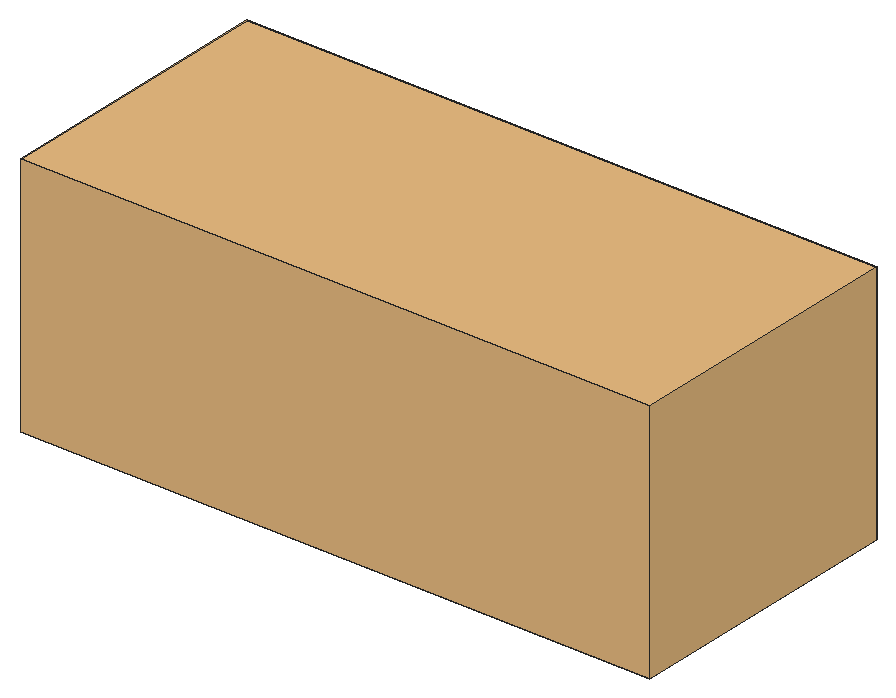
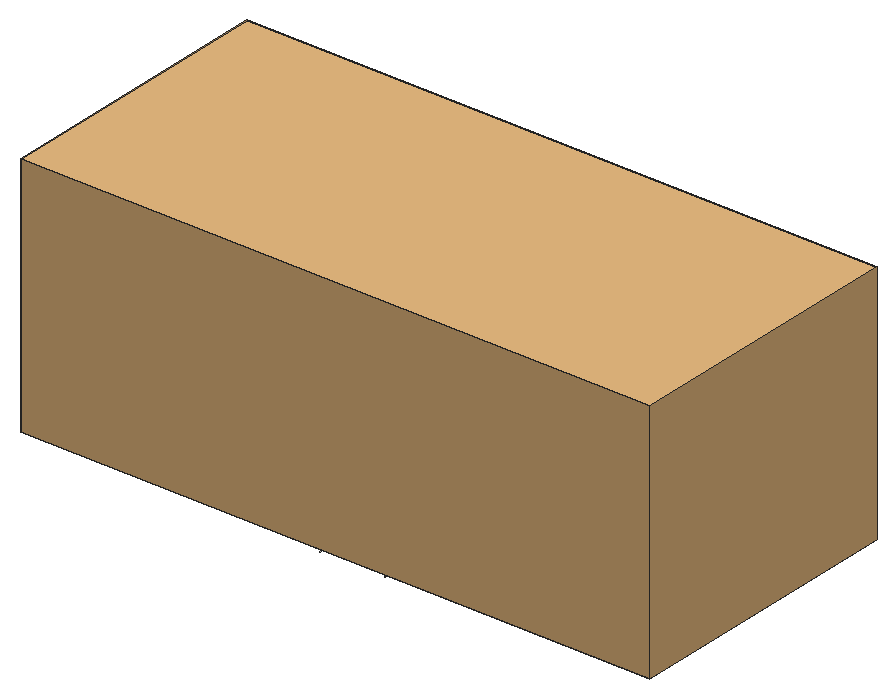
# SketchUp Ruby script. Lengths in inches.
U = 1.inch
M = Sketchup.active_model
def pt(a) = Geom::Point3d.new(a.map { |v| v * U })
def face(e, loops, mat)
  f = e.add_face(loops[0].map { |a| pt(a) })
  loops[1..].each { |l| e.add_face(l.map { |a| pt(a) }).erase! }
  f.material = f.back_material = mat if mat
  f
end
# faces: each face lists its corners as indices into pts; further lists are holes
def faces(e, pts, list, mat = nil) = list.each { |f| face(e, (f[0].is_a?(Array) ? f : [f]).map { |l| l.map { |i| pts[i] } }, mat) }
# xy, xz, yz: faces in a plane at the given z, y or x. An outline is a flat list of corners, or four numbers for a rectangle; further outlines are holes
def ring(l) = l.size == 4 ? [[l[0], l[1]], [l[2], l[1]], [l[2], l[3]], [l[0], l[3]]] : l.each_slice(2).to_a
def flat(e, list, mat, &to3) = list.each { |f| face(e, (f[0].is_a?(Array) ? f : [f]).map { |l| ring(l).map { |u, v| to3.(u, v) } }, mat) }
def xy(e, z, list, mat = nil) = flat(e, list, mat) { |x, y| [x, y, z] }
def xz(e, y, list, mat = nil) = flat(e, list, mat) { |x, z| [x, y, z] }
def yz(e, x, list, mat = nil) = flat(e, list, mat) { |y, z| [x, y, z] }
def lines(e, pts, list) = list.each { |a, b| e.add_line(pt(pts[a]), pt(pts[b])) }
# prism: a flat outline (further loops are holes) pulled along v
def prism(e, loops, v, mat = nil)
  f = face(e, loops, mat); d = Geom::Vector3d.new(v.map { |x| x * U })
  f.pushpull(f.normal.samedirection?(d) ? d.length : -d.length)
end
def box(e, o, s, mat = nil) = prism(e, [[o, [o[0] + s[0], o[1], o[2]], [o[0] + s[0], o[1] + s[1], o[2]], [o[0], o[1] + s[1], o[2]]]], [0, 0, s[2]], mat)
def at(x, y, z, deg = 0) = Geom::Transformation.translation(pt([x, y, z])) * Geom::Transformation.rotation(ORIGIN, Z_AXIS, deg.degrees)
def axes(o, x, y, z) = Geom::Transformation.new([*x, 0, *y, 0, *z, 0, *pt(o).to_a, 1])
def part(name) = M.definitions.add(name)
# library, detail: a bought-in or finely detailed component or shape, given as its bounding box
def library(name, o, s) = part(name).tap { |d| box(d.entities, o, s) }
def detail(e, o, s) = box(e.add_group.entities, o, s)
def put(e, d, t, mat = nil) = e.add_instance(d, t).tap { |i| i.material = mat if mat }
def group(e, t, mat = nil) = e.add_group.tap { |g| g.transformation = t; g.material = mat if mat }.entities
root = M.entities
M.materials.add("[Metal_Steel_Textured_White]").color = [191, 191, 191]
c1 = library("Land Rover Range Rover Sport",[-42.64,-96.16,0],[85.02,188.78,73.23])
xy(root,3.625,[[[147.359,164.396,134.847,169.578,143.617,178.348,148.799,165.836,148.641,165.764,148.487,165.682,148.339,165.59,148.198,165.489,148.063,165.378,147.936,165.259,147.817,165.132,147.706,164.998,147.605,164.856,147.513,164.708,147.431,164.555],[143.477,177.554,143.5,177.557,143.521,177.566,143.539,177.58,143.554,177.599,143.5625,177.62,143.566,177.643,143.5625,177.666,143.554,177.688,143.539,177.706,143.521,177.72,143.5,177.729,143.477,177.732,143.454,177.729,143.432,177.72,143.414,177.706,143.4,177.688,143.391,177.666,143.388,177.643,143.391,177.62,143.4,177.599,143.414,177.58,143.432,177.566,143.454,177.557],[139.514,173.592,139.537,173.595,139.559,173.604,139.577,173.618,139.591,173.637,139.6,173.658,139.603,173.681,139.6,173.704,139.591,173.725,139.577,173.744,139.559,173.758,139.537,173.767,139.514,173.77,139.491,173.767,139.47,173.758,139.451,173.744,139.4375,173.725,139.428,173.704,139.425,173.681,139.428,173.658,139.4375,173.637,139.451,173.618,139.47,173.604,139.491,173.595],[145.882,171.747,145.905,171.75,145.927,171.759,145.945,171.773,145.959,171.791,145.968,171.813,145.971,171.836,145.968,171.859,145.959,171.88,145.945,171.899,145.927,171.913,145.905,171.922,145.882,171.925,145.859,171.922,145.838,171.913,145.819,171.899,145.805,171.88,145.796,171.859,145.793,171.836,145.796,171.813,145.805,171.791,145.819,171.773,145.838,171.759,145.859,171.75],[141.495,175.573,141.518,175.576,141.54,175.585,141.558,175.599,141.572,175.618,141.581,175.639,141.584,175.662,141.581,175.685,141.572,175.707,141.558,175.725,141.54,175.739,141.518,175.748,141.495,175.751,141.472,175.748,141.451,175.739,141.433,175.725,141.418,175.707,141.41,175.685,141.407,175.662,141.41,175.639,141.418,175.618,141.433,175.599,141.451,175.585,141.472,175.576],[135.552,169.63,135.575,169.633,135.596,169.642,135.615,169.656,135.629,169.674,135.638,169.696,135.641,169.719,135.638,169.742,135.629,169.763,135.615,169.782,135.596,169.796,135.575,169.805,135.552,169.808,135.529,169.805,135.508,169.796,135.489,169.782,135.475,169.763,135.466,169.742,135.463,169.719,135.466,169.696,135.475,169.674,135.489,169.656,135.508,169.642,135.529,169.633],[148.288,165.939,148.311,165.942,148.332,165.951,148.351,165.965,148.365,165.984,148.374,166.005,148.377,166.028,148.374,166.051,148.365,166.073,148.351,166.091,148.332,166.105,148.311,166.114,148.288,166.117,148.265,166.114,148.243,166.105,148.225,166.091,148.211,166.073,148.202,166.051,148.199,166.028,148.202,166.005,148.211,165.984,148.225,165.965,148.243,165.951,148.265,165.942],[143.513,169.593,143.536,169.596,143.558,169.605,143.576,169.619,143.59,169.637,143.599,169.659,143.602,169.682,143.599,169.705,143.59,169.726,143.576,169.745,143.558,169.759,143.536,169.768,143.513,169.771,143.49,169.768,143.469,169.759,143.451,169.745,143.436,169.726,143.428,169.705,143.425,169.682,143.428,169.659,143.436,169.637,143.451,169.619,143.469,169.605,143.49,169.596],[137.533,171.611,137.556,171.614,137.578,171.623,137.596,171.637,137.61,171.655,137.619,171.677,137.622,171.7,137.619,171.723,137.61,171.744,137.596,171.763,137.578,171.777,137.556,171.786,137.533,171.789,137.51,171.786,137.489,171.777,137.47,171.763,137.456,171.744,137.447,171.723,137.444,171.7,137.447,171.677,137.456,171.655,137.47,171.637,137.489,171.623,137.51,171.614],[147.167,164.819,147.19,164.822,147.212,164.831,147.23,164.845,147.244,164.863,147.253,164.885,147.256,164.908,147.253,164.931,147.244,164.952,147.23,164.97,147.212,164.984,147.19,164.993,147.167,164.996,147.144,164.993,147.123,164.984,147.104,164.97,147.09,164.952,147.081,164.931,147.078,164.908,147.081,164.885,147.09,164.863,147.104,164.845,147.123,164.831,147.144,164.822],[144.679,174.651,144.702,174.654,144.724,174.663,144.742,174.677,144.756,174.695,144.765,174.717,144.768,174.74,144.765,174.763,144.756,174.784,144.742,174.802,144.724,174.817,144.702,174.825,144.679,174.828,144.656,174.825,144.635,174.817,144.617,174.802,144.602,174.784,144.594,174.763,144.591,174.74,144.594,174.717,144.602,174.695,144.617,174.677,144.635,174.663,144.656,174.654],[138.456,168.427,138.479,168.43,138.5,168.439,138.519,168.453,138.533,168.471,138.542,168.493,138.545,168.516,138.542,168.539,138.533,168.56,138.519,168.579,138.5,168.593,138.479,168.602,138.456,168.605,138.433,168.602,138.411,168.593,138.393,168.579,138.379,168.56,138.37,168.539,138.367,168.516,138.37,168.493,138.379,168.471,138.393,168.453,138.411,168.439,138.433,168.43],[141.36,167.224,141.383,167.227,141.404,167.236,141.422,167.25,141.437,167.269,141.445,167.29,141.448,167.313,141.445,167.336,141.437,167.358,141.422,167.376,141.404,167.39,141.383,167.399,141.36,167.402,141.337,167.399,141.315,167.39,141.297,167.376,141.283,167.358,141.274,167.336,141.271,167.313,141.274,167.29,141.283,167.269,141.297,167.25,141.315,167.236,141.337,167.227],[147.085,168.843,147.108,168.846,147.129,168.855,147.148,168.869,147.162,168.888,147.171,168.909,147.174,168.932,147.171,168.955,147.162,168.976,147.148,168.995,147.129,169.009,147.108,169.018,147.085,169.021,147.062,169.018,147.041,169.009,147.022,168.995,147.008,168.976,146.999,168.955,146.996,168.932,146.999,168.909,147.008,168.888,147.022,168.869,147.041,168.855,147.062,168.846],[144.263,166.021,144.286,166.024,144.308,166.033,144.326,166.047,144.34,166.066,144.349,166.087,144.352,166.11,144.349,166.133,144.34,166.155,144.326,166.173,144.308,166.187,144.286,166.196,144.263,166.199,144.24,166.196,144.219,166.187,144.2,166.173,144.186,166.155,144.177,166.133,144.174,166.11,144.177,166.087,144.186,166.066,144.2,166.047,144.219,166.033,144.24,166.024]],[[128.792,164.996,128.783,164.997,128.774,165.001,128.767,165.007,128.761,165.015,128.757,165.023,128.756,165.033,128.757,165.042,128.761,165.051,128.767,165.059,128.774,165.065,128.783,165.068,128.792,165.069,128.802,165.068,128.811,165.065,128.818,165.059,128.824,165.051,128.828,165.042,128.829,165.033,128.828,165.023,128.824,165.015,128.818,165.007,128.811,165.001,128.802,164.997],[128.792,165.013,128.798,165.014,128.802,165.016,128.807,165.019,128.81,165.023,128.812,165.028,128.8125,165.033,128.812,165.038,128.81,165.043,128.807,165.047,128.802,165.05,128.798,165.052,128.792,165.053,128.787,165.052,128.782,165.05,128.778,165.047,128.775,165.043,128.773,165.038,128.772,165.033,128.773,165.028,128.775,165.023,128.778,165.019,128.782,165.016,128.787,165.014]],[128.792,165.013,128.787,165.014,128.782,165.016,128.778,165.019,128.775,165.023,128.773,165.028,128.772,165.033,128.773,165.038,128.775,165.043,128.778,165.047,128.782,165.05,128.787,165.052,128.792,165.053,128.798,165.052,128.802,165.05,128.807,165.047,128.81,165.043,128.812,165.038,128.8125,165.033,128.812,165.028,128.81,165.023,128.807,165.019,128.802,165.016,128.798,165.014],[[148.799,165.836,143.617,178.348,156.019,178.348,150.836,165.836,150.673,165.898,150.507,165.948,150.337,165.988,150.165,166.016,149.992,166.033,149.818,166.039,149.644,166.033,149.471,166.016,149.299,165.988,149.129,165.948,148.962,165.898],[149.818,172.204,149.841,172.207,149.862,172.216,149.881,172.23,149.895,172.249,149.904,172.27,149.907,172.293,149.904,172.316,149.895,172.338,149.881,172.356,149.862,172.37,149.841,172.379,149.818,172.382,149.795,172.379,149.773,172.37,149.755,172.356,149.741,172.338,149.732,172.316,149.729,172.293,149.732,172.27,149.741,172.249,149.755,172.23,149.773,172.216,149.795,172.207],[154.219,174.956,154.242,174.959,154.263,174.968,154.282,174.982,154.296,175.001,154.305,175.022,154.308,175.045,154.305,175.068,154.296,175.09,154.282,175.108,154.263,175.122,154.242,175.131,154.219,175.134,154.196,175.131,154.174,175.122,154.156,175.108,154.142,175.09,154.133,175.068,154.13,175.045,154.133,175.022,154.142,175.001,154.156,174.982,154.174,174.968,154.196,174.959],[155.421,177.86,155.444,177.863,155.466,177.872,155.484,177.886,155.498,177.904,155.507,177.926,155.51,177.949,155.507,177.972,155.498,177.993,155.484,178.012,155.466,178.026,155.444,178.035,155.421,178.038,155.398,178.035,155.377,178.026,155.359,178.012,155.345,177.993,155.336,177.972,155.333,177.949,155.336,177.926,155.345,177.904,155.359,177.886,155.377,177.872,155.398,177.863],[144.214,177.86,144.237,177.863,144.259,177.872,144.277,177.886,144.291,177.904,144.3,177.926,144.303,177.949,144.3,177.972,144.291,177.993,144.277,178.012,144.259,178.026,144.237,178.035,144.214,178.038,144.191,178.035,144.17,178.026,144.151,178.012,144.137,177.993,144.128,177.972,144.125,177.949,144.128,177.926,144.137,177.904,144.151,177.886,144.17,177.872,144.191,177.863],[153.016,172.052,153.039,172.055,153.06,172.064,153.079,172.078,153.093,172.097,153.102,172.118,153.105,172.141,153.102,172.164,153.093,172.186,153.079,172.204,153.06,172.218,153.039,172.227,153.016,172.23,152.993,172.227,152.971,172.218,152.953,172.204,152.939,172.186,152.93,172.164,152.927,172.141,152.93,172.118,152.939,172.097,152.953,172.078,152.971,172.064,152.993,172.055],[147.016,177.86,147.039,177.863,147.061,177.872,147.079,177.886,147.093,177.904,147.102,177.926,147.105,177.949,147.102,177.972,147.093,177.993,147.079,178.012,147.061,178.026,147.039,178.035,147.016,178.038,146.993,178.035,146.972,178.026,146.953,178.012,146.939,177.993,146.93,177.972,146.927,177.949,146.93,177.926,146.939,177.904,146.953,177.886,146.972,177.872,146.993,177.863],[152.62,177.86,152.643,177.863,152.664,177.872,152.683,177.886,152.697,177.904,152.706,177.926,152.709,177.949,152.706,177.972,152.697,177.993,152.683,178.012,152.664,178.026,152.643,178.035,152.62,178.038,152.597,178.035,152.575,178.026,152.557,178.012,152.543,177.993,152.534,177.972,152.531,177.949,152.534,177.926,152.543,177.904,152.557,177.886,152.575,177.872,152.597,177.863],[145.417,174.956,145.44,174.959,145.462,174.968,145.48,174.982,145.494,175.001,145.503,175.022,145.506,175.045,145.503,175.068,145.494,175.09,145.48,175.108,145.462,175.122,145.44,175.131,145.417,175.134,145.394,175.131,145.373,175.122,145.354,175.108,145.34,175.09,145.331,175.068,145.328,175.045,145.331,175.022,145.34,175.001,145.354,174.982,145.373,174.968,145.394,174.959],[149.818,177.86,149.841,177.863,149.862,177.872,149.881,177.886,149.895,177.904,149.904,177.926,149.907,177.949,149.904,177.972,149.895,177.993,149.881,178.012,149.862,178.026,149.841,178.035,149.818,178.038,149.795,178.035,149.773,178.026,149.755,178.012,149.741,177.993,149.732,177.972,149.729,177.949,149.732,177.926,149.741,177.904,149.755,177.886,149.773,177.872,149.795,177.863],[147.823,169.149,147.846,169.152,147.867,169.161,147.886,169.175,147.9,169.193,147.909,169.215,147.912,169.238,147.909,169.261,147.9,169.282,147.886,169.3,147.867,169.315,147.846,169.323,147.823,169.326,147.8,169.323,147.778,169.315,147.76,169.3,147.746,169.282,147.737,169.261,147.734,169.238,147.737,169.215,147.746,169.193,147.76,169.175,147.778,169.161,147.8,169.152],[151.813,169.149,151.836,169.152,151.858,169.161,151.876,169.175,151.89,169.193,151.899,169.215,151.902,169.238,151.899,169.261,151.89,169.282,151.876,169.3,151.858,169.315,151.836,169.323,151.813,169.326,151.79,169.323,151.769,169.315,151.75,169.3,151.736,169.282,151.727,169.261,151.724,169.238,151.727,169.215,151.736,169.193,151.75,169.175,151.769,169.161,151.79,169.152],[146.62,172.052,146.643,172.055,146.664,172.064,146.683,172.078,146.697,172.097,146.706,172.118,146.709,172.141,146.706,172.164,146.697,172.186,146.683,172.204,146.664,172.218,146.643,172.227,146.62,172.23,146.597,172.227,146.575,172.218,146.557,172.204,146.543,172.186,146.534,172.164,146.531,172.141,146.534,172.118,146.543,172.097,146.557,172.078,146.575,172.064,146.597,172.055],[149.025,166.245,149.048,166.248,149.07,166.257,149.088,166.271,149.102,166.289,149.111,166.311,149.114,166.334,149.111,166.357,149.102,166.378,149.088,166.397,149.07,166.411,149.048,166.42,149.025,166.423,149.002,166.42,148.981,166.411,148.963,166.397,148.948,166.378,148.94,166.357,148.937,166.334,148.94,166.311,148.948,166.289,148.963,166.271,148.981,166.257,149.002,166.248],[150.61,166.245,150.633,166.248,150.655,166.257,150.673,166.271,150.6875,166.289,150.696,166.311,150.699,166.334,150.696,166.357,150.6875,166.378,150.673,166.397,150.655,166.411,150.633,166.42,150.61,166.423,150.587,166.42,150.566,166.411,150.547,166.397,150.533,166.378,150.524,166.357,150.521,166.334,150.524,166.311,150.533,166.289,150.547,166.271,150.566,166.257,150.587,166.248]],[[144.263,166.021,144.24,166.024,144.219,166.033,144.2,166.047,144.186,166.066,144.177,166.087,144.174,166.11,144.177,166.133,144.186,166.155,144.2,166.173,144.219,166.187,144.24,166.196,144.263,166.199,144.286,166.196,144.308,166.187,144.326,166.173,144.34,166.155,144.349,166.133,144.352,166.11,144.349,166.087,144.34,166.066,144.326,166.047,144.308,166.033,144.286,166.024],[144.263,166.022,144.286,166.025,144.307,166.034,144.326,166.048,144.339,166.066,144.348,166.088,144.351,166.11,144.348,166.133,144.339,166.154,144.326,166.172,144.307,166.186,144.286,166.195,144.263,166.198,144.241,166.195,144.219,166.186,144.201,166.172,144.187,166.154,144.178,166.133,144.175,166.11,144.178,166.088,144.187,166.066,144.201,166.048,144.219,166.034,144.241,166.025]],
  [[144.263,166.022,144.241,166.025,144.219,166.034,144.201,166.048,144.187,166.066,144.178,166.088,144.175,166.11,144.178,166.133,144.187,166.154,144.201,166.172,144.219,166.186,144.241,166.195,144.263,166.198,144.286,166.195,144.307,166.186,144.326,166.172,144.339,166.154,144.348,166.133,144.351,166.11,144.348,166.088,144.339,166.066,144.326,166.048,144.307,166.034,144.286,166.025],[144.263,166.074,144.273,166.075,144.282,166.079,144.289,166.084,144.295,166.092,144.299,166.101,144.3,166.11,144.299,166.12,144.295,166.129,144.289,166.136,144.282,166.142,144.273,166.146,144.263,166.147,144.254,166.146,144.245,166.142,144.237,166.136,144.232,166.129,144.228,166.12,144.227,166.11,144.228,166.101,144.232,166.092,144.237,166.084,144.245,166.079,144.254,166.075]],[[135.246,166.09,135.223,166.093,135.202,166.102,135.184,166.116,135.169,166.135,135.161,166.156,135.158,166.179,135.161,166.202,135.169,166.224,135.184,166.242,135.202,166.256,135.223,166.265,135.246,166.268,135.269,166.265,135.291,166.256,135.309,166.242,135.323,166.224,135.332,166.202,135.335,166.179,135.332,166.156,135.323,166.135,135.309,166.116,135.291,166.102,135.269,166.093],[135.246,166.091,135.269,166.094,135.29,166.103,135.309,166.117,135.323,166.135,135.331,166.156,135.334,166.179,135.331,166.202,135.323,166.223,135.309,166.241,135.29,166.255,135.269,166.264,135.246,166.267,135.224,166.264,135.202,166.255,135.184,166.241,135.17,166.223,135.161,166.202,135.159,166.179,135.161,166.156,135.17,166.135,135.184,166.117,135.202,166.103,135.224,166.094]],[[135.246,166.143,135.237,166.144,135.228,166.148,135.221,166.153,135.215,166.161,135.211,166.17,135.21,166.179,135.211,166.189,135.215,166.198,135.221,166.205,135.228,166.211,135.237,166.215,135.246,166.216,135.256,166.215,135.265,166.211,135.272,166.205,135.278,166.198,135.282,166.189,135.283,166.179,135.282,166.17,135.278,166.161,135.272,166.153,135.265,166.148,135.256,166.144],[135.246,166.159,135.252,166.16,135.256,166.162,135.261,166.165,135.264,166.169,135.266,166.174,135.266,166.184,135.264,166.189,135.261,166.193,135.256,166.197,135.252,166.198,135.246,166.199,135.236,166.197,135.232,166.193,135.229,166.189,135.227,166.184,135.226,166.179,135.227,166.174,135.229,166.169,135.232,166.165,135.236,166.162,135.241,166.16]],[135.246,166.159,135.241,166.16,135.236,166.162,135.232,166.165,135.229,166.169,135.227,166.174,135.226,166.179,135.227,166.184,135.229,166.189,135.232,166.193,135.236,166.197,135.246,166.199,135.252,166.198,135.256,166.197,135.261,166.193,135.264,166.189,135.266,166.184,135.266,166.174,135.264,166.169,135.261,166.165,135.256,166.162,135.252,166.16],[[134.448,166.256,134.425,166.259,134.404,166.268,134.385,166.282,134.371,166.3,134.362,166.322,134.359,166.345,134.362,166.368,134.371,166.389,134.385,166.407,134.404,166.422,134.425,166.43,134.448,166.433,134.471,166.43,134.492,166.422,134.511,166.407,134.525,166.389,134.534,166.368,134.537,166.345,134.534,166.322,134.525,166.3,134.511,166.282,134.492,166.268,134.471,166.259],[134.448,166.257,134.471,166.26,134.492,166.268,134.51,166.282,134.524,166.301,134.533,166.322,134.536,166.345,134.533,166.367,134.524,166.389,134.51,166.407,134.492,166.421,134.471,166.43,134.448,166.433,134.425,166.43,134.404,166.421,134.386,166.407,134.372,166.389,134.363,166.367,134.36,166.345,134.363,166.322,134.372,166.301,134.386,166.282,134.404,166.268,134.425,166.26]],
  [[134.448,166.308,134.439,166.309,134.43,166.313,134.422,166.319,134.416,166.326,134.413,166.335,134.411,166.345,134.413,166.354,134.416,166.363,134.422,166.37,134.43,166.376,134.439,166.38,134.448,166.381,134.457,166.38,134.466,166.376,134.474,166.37,134.48,166.363,134.483,166.354,134.485,166.345,134.483,166.335,134.48,166.326,134.474,166.319,134.466,166.313,134.457,166.309],[134.443,166.325,134.453,166.325,134.458,166.327,134.462,166.33,134.465,166.335,134.467,166.339,134.468,166.345,134.467,166.35,134.465,166.355,134.462,166.359,134.458,166.362,134.453,166.364,134.448,166.365,134.443,166.364,134.438,166.362,134.434,166.359,134.431,166.355,134.429,166.35,134.428,166.345,134.429,166.339,134.431,166.335,134.434,166.33,134.438,166.327]],[134.443,166.325,134.438,166.327,134.434,166.33,134.431,166.335,134.429,166.339,134.428,166.345,134.429,166.35,134.431,166.355,134.434,166.359,134.438,166.362,134.443,166.364,134.448,166.365,134.453,166.364,134.458,166.362,134.462,166.359,134.465,166.355,134.467,166.35,134.468,166.345,134.467,166.339,134.465,166.335,134.462,166.33,134.458,166.327,134.453,166.325],[[141.054,166.487,141.031,166.49,141.01,166.498,140.991,166.513,140.977,166.531,140.968,166.552,140.965,166.575,140.968,166.598,140.977,166.62,140.991,166.638,141.01,166.652,141.031,166.661,141.054,166.664,141.077,166.661,141.098,166.652,141.117,166.638,141.131,166.62,141.14,166.598,141.143,166.575,141.14,166.552,141.131,166.531,141.117,166.513,141.098,166.498,141.077,166.49],[141.054,166.488,141.077,166.491,141.098,166.499,141.116,166.513,141.13,166.531,141.139,166.553,141.142,166.575,141.139,166.598,141.13,166.619,141.116,166.638,141.098,166.652,141.077,166.66,141.054,166.663,141.031,166.66,141.01,166.652,140.992,166.638,140.978,166.619,140.969,166.598,140.966,166.575,140.969,166.553,140.978,166.531,140.992,166.513,141.01,166.499,141.031,166.491]],[[123.81,166.578,123.787,166.581,123.765,166.59,123.747,166.604,123.733,166.623,123.724,166.644,123.721,166.667,123.724,166.69,123.733,166.712,123.747,166.73,123.765,166.744,123.787,166.753,123.81,166.756,123.833,166.753,123.854,166.744,123.873,166.73,123.887,166.712,123.896,166.69,123.899,166.667,123.896,166.644,123.887,166.623,123.873,166.604,123.854,166.59,123.833,166.581],[123.81,166.579,123.833,166.582,123.854,166.591,123.872,166.605,123.886,166.623,123.895,166.644,123.898,166.667,123.895,166.69,123.886,166.711,123.872,166.729,123.854,166.743,123.833,166.752,123.81,166.755,123.787,166.752,123.766,166.743,123.748,166.729,123.734,166.711,123.725,166.69,123.722,166.667,123.725,166.644,123.734,166.623,123.748,166.605,123.766,166.591,123.787,166.582]],[[123.81,166.631,123.8,166.632,123.792,166.636,123.784,166.641,123.778,166.649,123.774,166.658,123.773,166.667,123.774,166.677,123.778,166.686,123.784,166.693,123.792,166.699,123.8,166.703,123.81,166.704,123.819,166.703,123.828,166.699,123.836,166.693,123.841,166.686,123.845,166.677,123.846,166.667,123.845,166.658,123.841,166.649,123.836,166.641,123.828,166.636,123.819,166.632],[123.81,166.647,123.815,166.648,123.82,166.65,123.824,166.653,123.827,166.657,123.829,166.662,123.83,166.667,123.829,166.672,123.827,166.677,123.824,166.681,123.82,166.685,123.815,166.687,123.805,166.687,123.8,166.685,123.796,166.681,123.793,166.677,123.791,166.672,123.79,166.667,123.791,166.662,123.793,166.657,123.796,166.653,123.8,166.65,123.805,166.648]],
  [123.81,166.647,123.805,166.648,123.8,166.65,123.796,166.653,123.793,166.657,123.791,166.662,123.79,166.667,123.791,166.672,123.793,166.677,123.796,166.681,123.8,166.685,123.805,166.687,123.815,166.687,123.82,166.685,123.824,166.681,123.827,166.677,123.829,166.672,123.83,166.667,123.829,166.662,123.827,166.657,123.824,166.653,123.82,166.65,123.815,166.648],[[141.36,167.224,141.337,167.227,141.315,167.236,141.297,167.25,141.283,167.269,141.274,167.29,141.271,167.313,141.274,167.336,141.283,167.358,141.297,167.376,141.315,167.39,141.337,167.399,141.36,167.402,141.383,167.399,141.404,167.39,141.422,167.376,141.437,167.358,141.445,167.336,141.448,167.313,141.445,167.29,141.437,167.269,141.422,167.25,141.404,167.236,141.383,167.227],[141.36,167.225,141.382,167.228,141.404,167.237,141.422,167.251,141.436,167.269,141.444,167.29,141.447,167.313,141.444,167.336,141.436,167.357,141.422,167.375,141.404,167.389,141.382,167.398,141.36,167.401,141.337,167.398,141.316,167.389,141.297,167.375,141.283,167.357,141.275,167.336,141.272,167.313,141.275,167.29,141.283,167.269,141.297,167.251,141.316,167.237,141.337,167.228]],[[141.36,167.276,141.35,167.278,141.341,167.281,141.334,167.287,141.328,167.295,141.324,167.304,141.323,167.313,141.324,167.323,141.328,167.331,141.334,167.339,141.341,167.345,141.35,167.348,141.36,167.35,141.369,167.348,141.378,167.345,141.385,167.339,141.391,167.331,141.395,167.323,141.396,167.313,141.395,167.304,141.391,167.295,141.385,167.287,141.378,167.281,141.369,167.278],[141.36,167.293,141.365,167.294,141.37,167.296,141.374,167.299,141.377,167.303,141.379,167.308,141.38,167.313,141.379,167.318,141.377,167.323,141.374,167.327,141.37,167.33,141.365,167.332,141.36,167.333,141.354,167.332,141.35,167.33,141.345,167.327,141.342,167.323,141.34,167.318,141.34,167.308,141.342,167.303,141.345,167.299,141.35,167.296,141.354,167.294]],[141.36,167.293,141.354,167.294,141.35,167.296,141.345,167.299,141.342,167.303,141.34,167.308,141.34,167.318,141.342,167.323,141.345,167.327,141.35,167.33,141.354,167.332,141.36,167.333,141.365,167.332,141.37,167.33,141.374,167.327,141.377,167.323,141.379,167.318,141.38,167.313,141.379,167.308,141.377,167.303,141.374,167.299,141.37,167.296,141.365,167.294],[[138.15,167.689,138.127,167.692,138.106,167.701,138.087,167.715,138.073,167.734,138.064,167.755,138.061,167.778,138.064,167.801,138.073,167.823,138.087,167.841,138.106,167.855,138.127,167.864,138.15,167.867,138.173,167.864,138.195,167.855,138.213,167.841,138.227,167.823,138.236,167.801,138.239,167.778,138.236,167.755,138.227,167.734,138.213,167.715,138.195,167.701,138.173,167.692],[138.15,167.69,138.173,167.693,138.194,167.702,138.212,167.716,138.226,167.734,138.235,167.755,138.238,167.778,138.235,167.801,138.226,167.822,138.212,167.84,138.194,167.854,138.173,167.863,138.15,167.866,138.127,167.863,138.106,167.854,138.088,167.84,138.074,167.822,138.065,167.801,138.062,167.778,138.065,167.755,138.074,167.734,138.088,167.716,138.106,167.702,138.127,167.693]],
  [[138.15,167.742,138.141,167.743,138.132,167.747,138.124,167.752,138.119,167.76,138.115,167.769,138.114,167.778,138.115,167.788,138.119,167.797,138.124,167.804,138.132,167.81,138.141,167.814,138.15,167.815,138.16,167.814,138.169,167.81,138.176,167.804,138.182,167.797,138.186,167.788,138.187,167.778,138.186,167.769,138.182,167.76,138.176,167.752,138.169,167.747,138.16,167.743],[138.15,167.758,138.155,167.759,138.16,167.761,138.164,167.764,138.168,167.768,138.17,167.778,138.168,167.788,138.16,167.796,138.155,167.798,138.145,167.798,138.14,167.796,138.136,167.792,138.133,167.788,138.131,167.783,138.13,167.778,138.131,167.773,138.133,167.768,138.136,167.764,138.14,167.761,138.145,167.759]],[138.15,167.758,138.145,167.759,138.14,167.761,138.136,167.764,138.133,167.768,138.131,167.773,138.13,167.778,138.131,167.783,138.133,167.788,138.136,167.792,138.14,167.796,138.145,167.798,138.155,167.798,138.16,167.796,138.168,167.788,138.17,167.778,138.168,167.768,138.164,167.764,138.16,167.761,138.155,167.759],[[128.792,168.255,128.769,168.258,128.748,168.267,128.73,168.281,128.715,168.299,128.707,168.321,128.704,168.344,128.707,168.367,128.715,168.388,128.73,168.406,128.748,168.421,128.769,168.429,128.792,168.432,128.815,168.429,128.837,168.421,128.855,168.406,128.869,168.388,128.878,168.367,128.881,168.344,128.878,168.321,128.869,168.299,128.855,168.281,128.837,168.267,128.815,168.258],[128.792,168.256,128.815,168.259,128.836,168.267,128.855,168.281,128.869,168.3,128.877,168.321,128.88,168.344,128.877,168.366,128.869,168.388,128.855,168.406,128.836,168.42,128.815,168.429,128.792,168.432,128.77,168.429,128.748,168.42,128.73,168.406,128.716,168.388,128.707,168.366,128.704,168.344,128.707,168.321,128.716,168.3,128.73,168.281,128.748,168.267,128.77,168.259]],[[128.792,168.307,128.783,168.308,128.774,168.312,128.767,168.318,128.761,168.325,128.757,168.334,128.756,168.344,128.757,168.353,128.761,168.362,128.767,168.369,128.774,168.375,128.783,168.379,128.792,168.38,128.802,168.379,128.811,168.375,128.818,168.369,128.824,168.362,128.828,168.353,128.829,168.344,128.828,168.334,128.824,168.325,128.818,168.318,128.811,168.312,128.802,168.308],[128.787,168.324,128.798,168.324,128.802,168.326,128.807,168.329,128.81,168.334,128.812,168.338,128.8125,168.344,128.812,168.349,128.81,168.354,128.807,168.358,128.802,168.361,128.798,168.363,128.792,168.364,128.787,168.363,128.782,168.361,128.778,168.358,128.775,168.354,128.773,168.349,128.772,168.344,128.773,168.338,128.775,168.334,128.778,168.329,128.782,168.326]],[128.787,168.324,128.782,168.326,128.778,168.329,128.775,168.334,128.773,168.338,128.772,168.344,128.773,168.349,128.775,168.354,128.778,168.358,128.782,168.361,128.787,168.363,128.792,168.364,128.798,168.363,128.802,168.361,128.807,168.358,128.81,168.354,128.812,168.349,128.8125,168.344,128.812,168.338,128.81,168.334,128.807,168.329,128.802,168.326,128.798,168.324],
  [[138.456,168.427,138.433,168.43,138.411,168.439,138.393,168.453,138.379,168.471,138.37,168.493,138.367,168.516,138.37,168.539,138.379,168.56,138.393,168.579,138.411,168.593,138.433,168.602,138.456,168.605,138.479,168.602,138.5,168.593,138.519,168.579,138.533,168.56,138.542,168.539,138.545,168.516,138.542,168.493,138.533,168.471,138.519,168.453,138.5,168.439,138.479,168.43],[138.456,168.428,138.479,168.431,138.5,168.44,138.518,168.454,138.532,168.472,138.541,168.493,138.544,168.516,138.541,168.539,138.532,168.56,138.518,168.578,138.5,168.592,138.479,168.601,138.456,168.604,138.433,168.601,138.412,168.592,138.394,168.578,138.38,168.56,138.371,168.539,138.368,168.516,138.371,168.493,138.38,168.472,138.394,168.454,138.412,168.44,138.433,168.431]],[[138.456,168.479,138.446,168.481,138.4375,168.484,138.43,168.49,138.424,168.498,138.42,168.506,138.419,168.516,138.42,168.525,138.424,168.534,138.43,168.542,138.4375,168.548,138.446,168.551,138.456,168.552,138.465,168.551,138.474,168.548,138.482,168.542,138.487,168.534,138.491,168.525,138.492,168.516,138.491,168.506,138.487,168.498,138.482,168.49,138.474,168.484,138.465,168.481],[138.456,168.496,138.461,168.497,138.466,168.499,138.47,168.502,138.473,168.506,138.475,168.511,138.476,168.516,138.475,168.521,138.473,168.526,138.47,168.53,138.466,168.533,138.461,168.535,138.456,168.536,138.451,168.535,138.446,168.533,138.442,168.53,138.438,168.526,138.436,168.521,138.436,168.511,138.438,168.506,138.442,168.502,138.446,168.499,138.451,168.497]],[138.456,168.496,138.451,168.497,138.446,168.499,138.442,168.502,138.438,168.506,138.436,168.511,138.436,168.521,138.438,168.526,138.442,168.53,138.446,168.533,138.451,168.535,138.456,168.536,138.461,168.535,138.466,168.533,138.47,168.53,138.473,168.526,138.475,168.521,138.476,168.516,138.475,168.511,138.473,168.506,138.47,168.502,138.466,168.499,138.461,168.497],[[135.246,168.892,135.223,168.895,135.202,168.904,135.184,168.918,135.169,168.937,135.161,168.958,135.158,168.981,135.161,169.004,135.169,169.025,135.184,169.044,135.202,169.058,135.223,169.067,135.246,169.07,135.269,169.067,135.291,169.058,135.309,169.044,135.323,169.025,135.332,169.004,135.335,168.981,135.332,168.958,135.323,168.937,135.309,168.918,135.291,168.904,135.269,168.895],[135.246,168.893,135.269,168.896,135.29,168.905,135.309,168.919,135.323,168.937,135.331,168.958,135.334,168.981,135.331,169.004,135.323,169.025,135.309,169.043,135.29,169.057,135.269,169.066,135.246,169.069,135.224,169.066,135.202,169.057,135.184,169.043,135.17,169.025,135.161,169.004,135.159,168.981,135.161,168.958,135.17,168.937,135.184,168.919,135.202,168.905,135.224,168.896]],[[135.246,168.944,135.237,168.946,135.228,168.949,135.221,168.955,135.215,168.963,135.211,168.972,135.21,168.981,135.211,168.99,135.215,168.999,135.221,169.007,135.228,169.013,135.237,169.016,135.246,169.018,135.256,169.016,135.265,169.013,135.272,169.007,135.278,168.999,135.282,168.99,135.283,168.981,135.282,168.972,135.278,168.963,135.272,168.955,135.265,168.949,135.256,168.946],[135.246,168.961,135.252,168.962,135.256,168.964,135.261,168.967,135.264,168.971,135.266,168.976,135.266,168.986,135.264,168.991,135.261,168.995,135.256,168.998,135.252,169,135.246,169.001,135.241,169,135.236,168.998,135.232,168.995,135.229,168.991,135.227,168.986,135.226,168.981,135.227,168.976,135.229,168.971,135.232,168.967,135.236,168.964,135.241,168.962]],
  [135.246,168.961,135.241,168.962,135.236,168.964,135.232,168.967,135.229,168.971,135.227,168.976,135.226,168.981,135.227,168.986,135.229,168.991,135.232,168.995,135.236,168.998,135.241,169,135.246,169.001,135.252,169,135.256,168.998,135.261,168.995,135.264,168.991,135.266,168.986,135.266,168.976,135.264,168.971,135.261,168.967,135.256,168.964,135.252,168.962],[[147.823,169.201,147.813,169.202,147.804,169.206,147.797,169.212,147.791,169.219,147.787,169.228,147.786,169.238,147.787,169.247,147.791,169.256,147.797,169.263,147.804,169.269,147.813,169.273,147.823,169.274,147.832,169.273,147.841,169.269,147.849,169.263,147.854,169.256,147.858,169.247,147.859,169.238,147.858,169.228,147.854,169.219,147.849,169.212,147.841,169.206,147.832,169.202],[147.818,169.218,147.828,169.218,147.833,169.22,147.837,169.223,147.84,169.228,147.842,169.232,147.843,169.238,147.842,169.243,147.84,169.248,147.837,169.252,147.833,169.255,147.828,169.257,147.818,169.257,147.8125,169.255,147.809,169.252,147.805,169.248,147.803,169.243,147.803,169.232,147.805,169.228,147.809,169.223,147.8125,169.22]],[147.818,169.218,147.8125,169.22,147.809,169.223,147.805,169.228,147.803,169.232,147.803,169.243,147.805,169.248,147.809,169.252,147.8125,169.255,147.818,169.257,147.828,169.257,147.833,169.255,147.837,169.252,147.84,169.248,147.842,169.243,147.843,169.238,147.842,169.232,147.84,169.228,147.837,169.223,147.833,169.22,147.828,169.218],[[134.448,169.275,134.439,169.276,134.43,169.28,134.422,169.286,134.416,169.293,134.413,169.302,134.411,169.312,134.413,169.321,134.416,169.33,134.422,169.338,134.43,169.343,134.439,169.347,134.448,169.348,134.457,169.347,134.466,169.343,134.474,169.338,134.48,169.33,134.483,169.321,134.485,169.312,134.483,169.302,134.48,169.293,134.474,169.286,134.466,169.28,134.457,169.276],[134.443,169.292,134.453,169.292,134.458,169.294,134.462,169.298,134.465,169.302,134.467,169.307,134.468,169.312,134.467,169.317,134.465,169.322,134.462,169.326,134.458,169.329,134.453,169.331,134.448,169.332,134.443,169.331,134.438,169.329,134.434,169.326,134.431,169.322,134.429,169.317,134.428,169.312,134.429,169.307,134.431,169.302,134.434,169.298,134.438,169.294]],[134.443,169.292,134.438,169.294,134.434,169.298,134.431,169.302,134.429,169.307,134.428,169.312,134.429,169.317,134.431,169.322,134.434,169.326,134.438,169.329,134.443,169.331,134.448,169.332,134.453,169.331,134.458,169.329,134.462,169.326,134.465,169.322,134.467,169.317,134.468,169.312,134.467,169.307,134.465,169.302,134.462,169.298,134.458,169.294,134.453,169.292],
  [[143.513,169.593,143.49,169.596,143.469,169.605,143.451,169.619,143.436,169.637,143.428,169.659,143.425,169.682,143.428,169.705,143.436,169.726,143.451,169.745,143.469,169.759,143.49,169.768,143.513,169.771,143.536,169.768,143.558,169.759,143.576,169.745,143.59,169.726,143.599,169.705,143.602,169.682,143.599,169.659,143.59,169.637,143.576,169.619,143.558,169.605,143.536,169.596],[143.513,169.594,143.536,169.597,143.557,169.606,143.576,169.62,143.59,169.638,143.598,169.659,143.601,169.682,143.598,169.705,143.59,169.726,143.576,169.744,143.557,169.758,143.536,169.767,143.513,169.77,143.491,169.767,143.469,169.758,143.451,169.744,143.437,169.726,143.428,169.705,143.425,169.682,143.428,169.659,143.437,169.638,143.451,169.62,143.469,169.606,143.491,169.597]],[[135.552,169.63,135.529,169.633,135.508,169.642,135.489,169.656,135.475,169.674,135.466,169.696,135.463,169.719,135.466,169.742,135.475,169.763,135.489,169.782,135.508,169.796,135.529,169.805,135.552,169.808,135.575,169.805,135.596,169.796,135.615,169.782,135.629,169.763,135.638,169.742,135.641,169.719,135.638,169.696,135.629,169.674,135.615,169.656,135.596,169.642,135.575,169.633],[135.552,169.631,135.575,169.634,135.596,169.643,135.614,169.656,135.628,169.675,135.637,169.696,135.64,169.719,135.637,169.741,135.628,169.763,135.614,169.781,135.596,169.795,135.575,169.804,135.552,169.807,135.529,169.804,135.508,169.795,135.49,169.781,135.476,169.763,135.467,169.741,135.464,169.719,135.467,169.696,135.476,169.675,135.49,169.656,135.508,169.643,135.529,169.634]],[[143.513,169.645,143.504,169.647,143.495,169.65,143.488,169.656,143.482,169.664,143.478,169.672,143.477,169.682,143.478,169.691,143.482,169.7,143.488,169.708,143.495,169.714,143.504,169.717,143.513,169.718,143.523,169.717,143.532,169.714,143.539,169.708,143.545,169.7,143.549,169.691,143.55,169.682,143.549,169.672,143.545,169.664,143.539,169.656,143.532,169.65,143.523,169.647],[143.513,169.662,143.519,169.663,143.523,169.665,143.528,169.668,143.531,169.672,143.533,169.677,143.533,169.687,143.531,169.692,143.528,169.696,143.523,169.699,143.519,169.701,143.513,169.702,143.508,169.701,143.503,169.699,143.499,169.696,143.496,169.692,143.494,169.687,143.493,169.682,143.494,169.677,143.496,169.672,143.499,169.668,143.503,169.665,143.508,169.663]],[143.513,169.662,143.508,169.663,143.503,169.665,143.499,169.668,143.496,169.672,143.494,169.677,143.493,169.682,143.494,169.687,143.496,169.692,143.499,169.696,143.503,169.699,143.508,169.701,143.513,169.702,143.519,169.701,143.523,169.699,143.528,169.696,143.531,169.692,143.533,169.687,143.533,169.677,143.531,169.672,143.528,169.668,143.523,169.665,143.519,169.663],[[135.552,169.682,135.543,169.683,135.534,169.687,135.526,169.693,135.52,169.7,135.517,169.709,135.515,169.719,135.517,169.728,135.52,169.737,135.526,169.745,135.534,169.75,135.543,169.754,135.552,169.755,135.561,169.754,135.57,169.75,135.578,169.745,135.584,169.737,135.587,169.728,135.589,169.719,135.587,169.709,135.584,169.7,135.578,169.693,135.57,169.687,135.561,169.683],[135.547,169.699,135.557,169.699,135.562,169.701,135.566,169.705,135.569,169.709,135.571,169.714,135.572,169.719,135.571,169.724,135.569,169.729,135.566,169.733,135.562,169.736,135.557,169.738,135.552,169.739,135.547,169.738,135.542,169.736,135.538,169.733,135.535,169.729,135.533,169.724,135.532,169.719,135.533,169.714,135.535,169.709,135.538,169.705,135.542,169.701]],
  [135.547,169.699,135.542,169.701,135.538,169.705,135.535,169.709,135.533,169.714,135.532,169.719,135.533,169.724,135.535,169.729,135.538,169.733,135.542,169.736,135.547,169.738,135.552,169.739,135.557,169.738,135.562,169.736,135.566,169.733,135.569,169.729,135.571,169.724,135.572,169.719,135.571,169.714,135.569,169.709,135.566,169.705,135.562,169.701,135.557,169.699],[[124.428,169.816,124.405,169.819,124.384,169.828,124.365,169.842,124.351,169.861,124.342,169.882,124.339,169.905,124.342,169.928,124.351,169.949,124.365,169.968,124.384,169.982,124.405,169.991,124.428,169.994,124.451,169.991,124.473,169.982,124.491,169.968,124.505,169.949,124.514,169.928,124.517,169.905,124.514,169.882,124.505,169.861,124.491,169.842,124.473,169.828,124.451,169.819],[124.428,169.817,124.451,169.82,124.472,169.829,124.49,169.843,124.504,169.861,124.513,169.882,124.516,169.905,124.513,169.928,124.504,169.949,124.49,169.967,124.472,169.981,124.451,169.99,124.428,169.993,124.405,169.99,124.384,169.981,124.366,169.967,124.352,169.949,124.343,169.928,124.34,169.905,124.343,169.882,124.352,169.861,124.366,169.843,124.384,169.829,124.405,169.82]],[[124.428,169.817,124.405,169.82,124.384,169.829,124.366,169.843,124.352,169.861,124.343,169.882,124.34,169.905,124.343,169.928,124.352,169.949,124.366,169.967,124.384,169.981,124.405,169.99,124.428,169.993,124.451,169.99,124.472,169.981,124.49,169.967,124.504,169.949,124.513,169.928,124.516,169.905,124.513,169.882,124.504,169.861,124.49,169.843,124.472,169.829,124.451,169.82],[124.428,169.868,124.438,169.87,124.447,169.873,124.454,169.879,124.46,169.887,124.464,169.896,124.465,169.905,124.464,169.914,124.46,169.923,124.454,169.931,124.447,169.937,124.438,169.94,124.428,169.942,124.419,169.94,124.41,169.937,124.402,169.931,124.397,169.923,124.393,169.914,124.392,169.905,124.393,169.896,124.397,169.887,124.402,169.879,124.41,169.873,124.419,169.87]],[[131.448,170.518,131.439,170.519,131.43,170.523,131.422,170.528,131.416,170.536,131.413,170.545,131.411,170.554,131.413,170.564,131.416,170.573,131.422,170.58,131.43,170.586,131.439,170.59,131.448,170.591,131.458,170.59,131.466,170.586,131.474,170.58,131.48,170.573,131.483,170.564,131.485,170.554,131.483,170.545,131.48,170.536,131.474,170.528,131.466,170.523,131.458,170.519],[131.448,170.534,131.453,170.535,131.458,170.537,131.462,170.54,131.465,170.544,131.467,170.549,131.468,170.554,131.467,170.56,131.465,170.564,131.462,170.568,131.458,170.572,131.453,170.574,131.443,170.574,131.438,170.572,131.434,170.568,131.431,170.564,131.429,170.56,131.428,170.554,131.429,170.549,131.431,170.544,131.434,170.54,131.438,170.537,131.443,170.535]],[131.448,170.534,131.443,170.535,131.438,170.537,131.434,170.54,131.431,170.544,131.429,170.549,131.428,170.554,131.429,170.56,131.431,170.564,131.434,170.568,131.438,170.572,131.443,170.574,131.453,170.574,131.458,170.572,131.462,170.568,131.465,170.564,131.467,170.56,131.468,170.554,131.467,170.549,131.465,170.544,131.462,170.54,131.458,170.537,131.453,170.535],
  [[137.533,171.663,137.524,171.664,137.515,171.668,137.507,171.674,137.501,171.682,137.498,171.69,137.497,171.7,137.498,171.709,137.501,171.718,137.507,171.726,137.515,171.732,137.524,171.735,137.533,171.736,137.543,171.735,137.551,171.732,137.559,171.726,137.565,171.718,137.568,171.709,137.57,171.7,137.568,171.69,137.565,171.682,137.559,171.674,137.551,171.668,137.543,171.664],[137.533,171.68,137.538,171.681,137.543,171.683,137.547,171.686,137.55,171.69,137.552,171.695,137.553,171.7,137.552,171.705,137.55,171.71,137.547,171.714,137.543,171.717,137.538,171.719,137.533,171.72,137.528,171.719,137.523,171.717,137.519,171.714,137.516,171.71,137.514,171.705,137.513,171.7,137.514,171.695,137.516,171.69,137.519,171.686,137.523,171.683,137.528,171.681]],[137.533,171.68,137.528,171.681,137.523,171.683,137.519,171.686,137.516,171.69,137.514,171.695,137.513,171.7,137.514,171.705,137.516,171.71,137.519,171.714,137.523,171.717,137.528,171.719,137.533,171.72,137.538,171.719,137.543,171.717,137.547,171.714,137.55,171.71,137.552,171.705,137.553,171.7,137.552,171.695,137.55,171.69,137.547,171.686,137.543,171.683,137.538,171.681],[[145.882,171.747,145.859,171.75,145.838,171.759,145.819,171.773,145.805,171.791,145.796,171.813,145.793,171.836,145.796,171.859,145.805,171.88,145.819,171.899,145.838,171.913,145.859,171.922,145.882,171.925,145.905,171.922,145.927,171.913,145.945,171.899,145.959,171.88,145.968,171.859,145.971,171.836,145.968,171.813,145.959,171.791,145.945,171.773,145.927,171.759,145.905,171.75],[145.882,171.748,145.905,171.751,145.926,171.76,145.944,171.774,145.958,171.792,145.967,171.813,145.97,171.836,145.967,171.859,145.958,171.88,145.944,171.898,145.926,171.912,145.905,171.921,145.882,171.924,145.859,171.921,145.838,171.912,145.82,171.898,145.806,171.88,145.797,171.859,145.794,171.836,145.797,171.813,145.806,171.792,145.82,171.774,145.838,171.76,145.859,171.751]],[[128.448,171.76,128.439,171.762,128.43,171.765,128.422,171.771,128.416,171.779,128.413,171.788,128.411,171.797,128.413,171.806,128.416,171.815,128.422,171.823,128.43,171.829,128.439,171.832,128.448,171.834,128.458,171.832,128.466,171.829,128.474,171.823,128.48,171.815,128.483,171.806,128.485,171.797,128.483,171.788,128.48,171.779,128.474,171.771,128.466,171.765,128.458,171.762],[128.448,171.777,128.453,171.778,128.458,171.78,128.462,171.783,128.465,171.787,128.467,171.792,128.468,171.797,128.467,171.802,128.465,171.807,128.462,171.811,128.458,171.814,128.453,171.816,128.448,171.817,128.443,171.816,128.438,171.814,128.434,171.811,128.431,171.807,128.429,171.802,128.428,171.797,128.429,171.792,128.431,171.787,128.434,171.783,128.438,171.78,128.443,171.778]],[128.448,171.777,128.443,171.778,128.438,171.78,128.434,171.783,128.431,171.787,128.429,171.792,128.428,171.797,128.429,171.802,128.431,171.807,128.434,171.811,128.438,171.814,128.443,171.816,128.448,171.817,128.453,171.816,128.458,171.814,128.462,171.811,128.465,171.807,128.467,171.802,128.468,171.797,128.467,171.792,128.465,171.787,128.462,171.783,128.458,171.78,128.453,171.778],
  [[146.62,172.052,146.597,172.055,146.575,172.064,146.557,172.078,146.543,172.097,146.534,172.118,146.531,172.141,146.534,172.164,146.543,172.186,146.557,172.204,146.575,172.218,146.597,172.227,146.62,172.23,146.643,172.227,146.664,172.218,146.683,172.204,146.697,172.186,146.706,172.164,146.709,172.141,146.706,172.118,146.697,172.097,146.683,172.078,146.664,172.064,146.643,172.055],[146.62,172.053,146.643,172.056,146.664,172.065,146.682,172.079,146.696,172.097,146.705,172.119,146.708,172.141,146.705,172.164,146.696,172.185,146.682,172.203,146.664,172.217,146.643,172.226,146.62,172.229,146.597,172.226,146.576,172.217,146.558,172.203,146.544,172.185,146.535,172.164,146.532,172.141,146.535,172.119,146.544,172.097,146.558,172.079,146.576,172.065,146.597,172.056]],[[136.852,172.059,136.829,172.062,136.807,172.071,136.789,172.085,136.775,172.103,136.766,172.124,136.763,172.147,136.766,172.17,136.775,172.192,136.789,172.21,136.807,172.224,136.829,172.233,136.852,172.236,136.875,172.233,136.896,172.224,136.914,172.21,136.929,172.192,136.9375,172.17,136.941,172.147,136.9375,172.124,136.929,172.103,136.914,172.085,136.896,172.071,136.875,172.062],[136.852,172.06,136.874,172.0625,136.896,172.071,136.914,172.085,136.928,172.104,136.937,172.125,136.94,172.147,136.937,172.17,136.928,172.191,136.914,172.21,136.896,172.224,136.874,172.232,136.852,172.235,136.829,172.232,136.808,172.224,136.789,172.21,136.775,172.191,136.767,172.17,136.764,172.147,136.767,172.125,136.775,172.104,136.789,172.085,136.808,172.071,136.829,172.0625]],[[125.448,173.003,125.439,173.004,125.43,173.008,125.422,173.014,125.416,173.021,125.413,173.03,125.412,173.04,125.413,173.049,125.416,173.058,125.422,173.065,125.43,173.071,125.439,173.075,125.448,173.076,125.458,173.075,125.466,173.071,125.474,173.065,125.48,173.058,125.483,173.049,125.485,173.04,125.483,173.03,125.48,173.021,125.474,173.014,125.466,173.008,125.458,173.004],[125.443,173.02,125.453,173.02,125.458,173.022,125.462,173.025,125.465,173.03,125.467,173.034,125.468,173.04,125.467,173.045,125.465,173.05,125.462,173.054,125.458,173.057,125.453,173.059,125.448,173.06,125.443,173.059,125.438,173.057,125.434,173.054,125.431,173.05,125.429,173.045,125.428,173.04,125.429,173.034,125.431,173.03,125.434,173.025,125.438,173.022]],[125.443,173.02,125.438,173.022,125.434,173.025,125.431,173.03,125.429,173.034,125.428,173.04,125.429,173.045,125.431,173.05,125.434,173.054,125.438,173.057,125.443,173.059,125.448,173.06,125.453,173.059,125.458,173.057,125.462,173.054,125.465,173.05,125.467,173.045,125.468,173.04,125.467,173.034,125.465,173.03,125.462,173.025,125.458,173.022,125.453,173.02],[[125.754,173.689,125.731,173.692,125.71,173.701,125.691,173.715,125.678,173.733,125.669,173.755,125.666,173.777,125.669,173.8,125.678,173.821,125.691,173.839,125.71,173.853,125.731,173.862,125.754,173.865,125.776,173.862,125.798,173.853,125.816,173.839,125.83,173.821,125.839,173.8,125.842,173.777,125.839,173.755,125.83,173.733,125.816,173.715,125.798,173.701,125.776,173.692],[125.754,173.741,125.763,173.742,125.772,173.746,125.78,173.751,125.785,173.759,125.789,173.768,125.79,173.777,125.789,173.787,125.785,173.796,125.78,173.803,125.772,173.809,125.763,173.8125,125.754,173.814,125.744,173.8125,125.735,173.809,125.728,173.803,125.722,173.796,125.718,173.787,125.717,173.777,125.718,173.768,125.722,173.759,125.728,173.751,125.735,173.746,125.744,173.742]],
  [[131.439,174.644,131.416,174.647,131.395,174.656,131.376,174.67,131.362,174.689,131.353,174.71,131.35,174.733,131.353,174.756,131.362,174.778,131.376,174.796,131.395,174.81,131.416,174.819,131.439,174.822,131.462,174.819,131.483,174.81,131.502,174.796,131.516,174.778,131.525,174.756,131.528,174.733,131.525,174.71,131.516,174.689,131.502,174.67,131.483,174.656,131.462,174.647],[131.439,174.645,131.462,174.648,131.483,174.657,131.501,174.671,131.515,174.689,131.524,174.71,131.527,174.733,131.524,174.756,131.515,174.777,131.501,174.795,131.483,174.809,131.462,174.818,131.439,174.821,131.416,174.818,131.395,174.809,131.377,174.795,131.363,174.777,131.354,174.756,131.351,174.733,131.354,174.71,131.363,174.689,131.377,174.671,131.395,174.657,131.416,174.648]],[[144.679,174.652,144.657,174.655,144.635,174.663,144.617,174.677,144.603,174.696,144.595,174.717,144.592,174.74,144.595,174.762,144.603,174.784,144.617,174.802,144.635,174.816,144.657,174.824,144.679,174.827,144.702,174.824,144.723,174.816,144.742,174.802,144.756,174.784,144.764,174.762,144.767,174.74,144.764,174.717,144.756,174.696,144.742,174.677,144.723,174.663,144.702,174.655],[144.679,174.703,144.689,174.704,144.698,174.708,144.705,174.714,144.711,174.721,144.715,174.73,144.716,174.74,144.715,174.749,144.711,174.758,144.705,174.765,144.698,174.771,144.689,174.775,144.679,174.776,144.67,174.775,144.661,174.771,144.654,174.765,144.648,174.758,144.644,174.749,144.643,174.74,144.644,174.73,144.648,174.721,144.654,174.714,144.661,174.708,144.67,174.704]],[[144.679,174.703,144.67,174.704,144.661,174.708,144.654,174.714,144.648,174.721,144.644,174.73,144.643,174.74,144.644,174.749,144.648,174.758,144.654,174.765,144.661,174.771,144.67,174.775,144.679,174.776,144.689,174.775,144.698,174.771,144.705,174.765,144.711,174.758,144.715,174.749,144.716,174.74,144.715,174.73,144.711,174.721,144.705,174.714,144.698,174.708,144.689,174.704],[144.674,174.72,144.685,174.72,144.689,174.722,144.694,174.725,144.697,174.73,144.699,174.734,144.699,174.745,144.697,174.75,144.694,174.754,144.689,174.757,144.685,174.759,144.679,174.76,144.674,174.759,144.669,174.757,144.665,174.754,144.662,174.75,144.66,174.745,144.659,174.74,144.66,174.734,144.662,174.73,144.665,174.725,144.669,174.722]],[[141.495,175.573,141.472,175.576,141.451,175.585,141.433,175.599,141.418,175.618,141.41,175.639,141.407,175.662,141.41,175.685,141.418,175.707,141.433,175.725,141.451,175.739,141.472,175.748,141.495,175.751,141.518,175.748,141.54,175.739,141.558,175.725,141.572,175.707,141.581,175.685,141.584,175.662,141.581,175.639,141.572,175.618,141.558,175.599,141.54,175.585,141.518,175.576],[141.495,175.574,141.518,175.577,141.539,175.586,141.558,175.6,141.572,175.618,141.58,175.639,141.583,175.662,141.58,175.685,141.572,175.706,141.558,175.724,141.539,175.738,141.518,175.747,141.495,175.75,141.473,175.747,141.452,175.738,141.433,175.724,141.419,175.706,141.411,175.685,141.408,175.662,141.411,175.639,141.419,175.618,141.433,175.6,141.452,175.586,141.473,175.577]],[[141.495,175.574,141.473,175.577,141.452,175.586,141.433,175.6,141.419,175.618,141.411,175.639,141.408,175.662,141.411,175.685,141.419,175.706,141.433,175.724,141.452,175.738,141.473,175.747,141.495,175.75,141.518,175.747,141.539,175.738,141.558,175.724,141.572,175.706,141.58,175.685,141.583,175.662,141.58,175.639,141.572,175.618,141.558,175.6,141.539,175.586,141.518,175.577],[141.495,175.626,141.505,175.627,141.514,175.63,141.521,175.636,141.527,175.644,141.531,175.653,141.532,175.662,141.531,175.672,141.527,175.68,141.521,175.688,141.514,175.694,141.505,175.698,141.495,175.699,141.486,175.698,141.477,175.694,141.47,175.688,141.464,175.68,141.46,175.672,141.459,175.662,141.46,175.653,141.464,175.644,141.47,175.636,141.477,175.63,141.486,175.627]],
  [141.495,175.642,141.49,175.643,141.485,175.645,141.481,175.648,141.478,175.652,141.476,175.657,141.476,175.667,141.478,175.672,141.481,175.676,141.485,175.679,141.49,175.681,141.495,175.682,141.501,175.681,141.505,175.679,141.51,175.676,141.513,175.672,141.515,175.667,141.515,175.657,141.513,175.652,141.51,175.648,141.505,175.645,141.501,175.643],[[141.048,176.255,141.025,176.258,141.003,176.267,140.985,176.281,140.971,176.299,140.962,176.321,140.959,176.344,140.962,176.367,140.971,176.388,140.985,176.407,141.003,176.421,141.025,176.43,141.048,176.433,141.071,176.43,141.092,176.421,141.111,176.407,141.125,176.388,141.134,176.367,141.137,176.344,141.134,176.321,141.125,176.299,141.111,176.281,141.092,176.267,141.071,176.258],[141.048,176.256,141.071,176.259,141.092,176.268,141.11,176.282,141.124,176.3,141.133,176.321,141.136,176.344,141.133,176.366,141.124,176.388,141.11,176.406,141.092,176.42,141.071,176.429,141.048,176.432,141.025,176.429,141.004,176.42,140.986,176.406,140.972,176.388,140.963,176.366,140.96,176.344,140.963,176.321,140.972,176.3,140.986,176.282,141.004,176.268,141.025,176.259]],[[127.249,176.626,127.226,176.629,127.205,176.638,127.186,176.652,127.172,176.67,127.163,176.692,127.16,176.715,127.163,176.738,127.172,176.759,127.186,176.778,127.205,176.792,127.226,176.801,127.249,176.804,127.272,176.801,127.293,176.792,127.312,176.778,127.326,176.759,127.335,176.738,127.338,176.715,127.335,176.692,127.326,176.67,127.312,176.652,127.293,176.638,127.272,176.629],[127.249,176.627,127.272,176.63,127.293,176.639,127.311,176.653,127.325,176.671,127.334,176.692,127.337,176.715,127.334,176.738,127.325,176.759,127.311,176.777,127.293,176.791,127.272,176.8,127.249,176.803,127.226,176.8,127.205,176.791,127.187,176.777,127.173,176.759,127.164,176.738,127.161,176.715,127.164,176.692,127.173,176.671,127.187,176.653,127.205,176.639,127.226,176.63]],[[133.78,176.985,133.757,176.988,133.736,176.997,133.717,177.011,133.703,177.03,133.694,177.051,133.691,177.074,133.694,177.097,133.703,177.119,133.717,177.137,133.736,177.151,133.757,177.16,133.78,177.163,133.803,177.16,133.825,177.151,133.843,177.137,133.857,177.119,133.866,177.097,133.869,177.074,133.866,177.051,133.857,177.03,133.843,177.011,133.825,176.997,133.803,176.988],[133.78,176.986,133.803,176.989,133.824,176.998,133.842,177.012,133.856,177.03,133.865,177.051,133.868,177.074,133.865,177.097,133.856,177.118,133.842,177.136,133.824,177.15,133.803,177.159,133.78,177.162,133.757,177.159,133.736,177.15,133.718,177.136,133.704,177.118,133.695,177.097,133.692,177.074,133.695,177.051,133.704,177.03,133.718,177.012,133.736,176.998,133.757,176.989]],[[133.78,177.038,133.771,177.039,133.762,177.042,133.754,177.048,133.748,177.056,133.745,177.065,133.743,177.074,133.745,177.084,133.748,177.092,133.754,177.1,133.762,177.106,133.771,177.11,133.78,177.111,133.79,177.11,133.798,177.106,133.806,177.1,133.812,177.092,133.815,177.084,133.817,177.074,133.815,177.065,133.812,177.056,133.806,177.048,133.798,177.042,133.79,177.039],[133.78,177.054,133.785,177.055,133.79,177.057,133.794,177.06,133.797,177.064,133.799,177.069,133.8,177.074,133.799,177.079,133.797,177.084,133.794,177.088,133.79,177.091,133.785,177.093,133.78,177.094,133.775,177.093,133.77,177.091,133.766,177.088,133.763,177.084,133.761,177.079,133.76,177.074,133.761,177.069,133.763,177.064,133.766,177.06,133.77,177.057,133.775,177.055]],
  [133.78,177.054,133.775,177.055,133.77,177.057,133.766,177.06,133.763,177.064,133.761,177.069,133.76,177.074,133.761,177.079,133.763,177.084,133.766,177.088,133.77,177.091,133.775,177.093,133.78,177.094,133.785,177.093,133.79,177.091,133.794,177.088,133.797,177.084,133.799,177.079,133.8,177.074,133.799,177.069,133.797,177.064,133.794,177.06,133.79,177.057,133.785,177.055],[[144.214,177.86,144.191,177.863,144.17,177.872,144.151,177.886,144.137,177.904,144.128,177.926,144.125,177.949,144.128,177.972,144.137,177.993,144.151,178.012,144.17,178.026,144.191,178.035,144.214,178.038,144.237,178.035,144.259,178.026,144.277,178.012,144.291,177.993,144.3,177.972,144.303,177.949,144.3,177.926,144.291,177.904,144.277,177.886,144.259,177.872,144.237,177.863],[144.214,177.861,144.237,177.864,144.258,177.873,144.276,177.887,144.29,177.905,144.299,177.926,144.302,177.949,144.299,177.972,144.29,177.993,144.276,178.011,144.258,178.025,144.237,178.034,144.214,178.037,144.192,178.034,144.17,178.025,144.152,178.011,144.138,177.993,144.129,177.972,144.126,177.949,144.129,177.926,144.138,177.905,144.152,177.887,144.17,177.873,144.192,177.864]],[[147.016,177.86,146.993,177.863,146.972,177.872,146.953,177.886,146.939,177.904,146.93,177.926,146.927,177.949,146.93,177.972,146.939,177.993,146.953,178.012,146.972,178.026,146.993,178.035,147.016,178.038,147.039,178.035,147.061,178.026,147.079,178.012,147.093,177.993,147.102,177.972,147.105,177.949,147.102,177.926,147.093,177.904,147.079,177.886,147.061,177.872,147.039,177.863],[147.016,177.861,147.039,177.864,147.06,177.873,147.078,177.887,147.092,177.905,147.101,177.926,147.104,177.949,147.101,177.972,147.092,177.993,147.078,178.011,147.06,178.025,147.039,178.034,147.016,178.037,146.993,178.034,146.972,178.025,146.954,178.011,146.94,177.993,146.931,177.972,146.928,177.949,146.931,177.926,146.94,177.905,146.954,177.887,146.972,177.873,146.993,177.864]],[149.818,177.86,149.795,177.863,149.773,177.872,149.755,177.886,149.741,177.904,149.732,177.926,149.729,177.949,149.732,177.972,149.741,177.993,149.755,178.012,149.773,178.026,149.795,178.035,149.818,178.038,149.818,178.037,149.795,178.034,149.774,178.025,149.756,178.011,149.742,177.993,149.733,177.972,149.73,177.949,149.733,177.926,149.742,177.905,149.756,177.887,149.774,177.873,149.795,177.864,149.818,177.861],[149.818,177.861,149.795,177.864,149.774,177.873,149.756,177.887,149.742,177.905,149.733,177.926,149.73,177.949,149.733,177.972,149.742,177.993,149.756,178.011,149.774,178.025,149.795,178.034,149.818,178.037,149.818,177.985,149.808,177.984,149.8,177.981,149.792,177.975,149.786,177.967,149.783,177.958,149.781,177.949,149.783,177.939,149.786,177.931,149.792,177.923,149.8,177.917,149.808,177.914,149.818,177.912],
  [149.818,177.912,149.808,177.914,149.8,177.917,149.792,177.923,149.786,177.931,149.783,177.939,149.781,177.949,149.783,177.958,149.786,177.967,149.792,177.975,149.8,177.981,149.808,177.984,149.818,177.985,149.818,177.969,149.813,177.968,149.808,177.966,149.804,177.963,149.801,177.959,149.799,177.954,149.798,177.949,149.799,177.944,149.801,177.939,149.804,177.935,149.808,177.932,149.813,177.93,149.818,177.929],[[143.884,178.711,143.874,178.712,143.865,178.716,143.858,178.721,143.852,178.729,143.848,178.738,143.847,178.747,143.848,178.757,143.852,178.766,143.858,178.773,143.865,178.779,143.874,178.783,143.884,178.784,143.893,178.783,143.902,178.779,143.909,178.773,143.915,178.766,143.919,178.757,143.92,178.747,143.919,178.738,143.915,178.729,143.909,178.721,143.902,178.716,143.893,178.712],[143.884,178.727,143.889,178.728,143.894,178.73,143.898,178.733,143.901,178.737,143.903,178.742,143.904,178.747,143.903,178.752,143.901,178.757,143.898,178.761,143.894,178.765,143.889,178.767,143.878,178.767,143.874,178.765,143.869,178.761,143.866,178.757,143.864,178.752,143.864,178.742,143.866,178.737,143.869,178.733,143.874,178.73,143.878,178.728]],[149.818,178.711,149.808,178.712,149.8,178.716,149.792,178.721,149.786,178.729,149.783,178.738,149.781,178.747,149.783,178.757,149.786,178.766,149.792,178.773,149.8,178.779,149.808,178.783,149.818,178.784,149.818,178.767,149.813,178.767,149.808,178.765,149.804,178.761,149.801,178.757,149.799,178.752,149.798,178.747,149.799,178.742,149.801,178.737,149.804,178.733,149.808,178.73,149.813,178.728,149.818,178.727],[143.884,178.727,143.878,178.728,143.874,178.73,143.869,178.733,143.866,178.737,143.864,178.742,143.864,178.752,143.866,178.757,143.869,178.761,143.874,178.765,143.878,178.767,143.889,178.767,143.894,178.765,143.898,178.761,143.901,178.757,143.903,178.752,143.904,178.747,143.903,178.742,143.901,178.737,143.898,178.733,143.894,178.73,143.889,178.728]],"[Metal_Steel_Textured_White]")
put(root,c1,axes([148.15,165.58,3.625],[0,0.3052,0],[-0.3052,0,0],[0,0,0.3052]))
